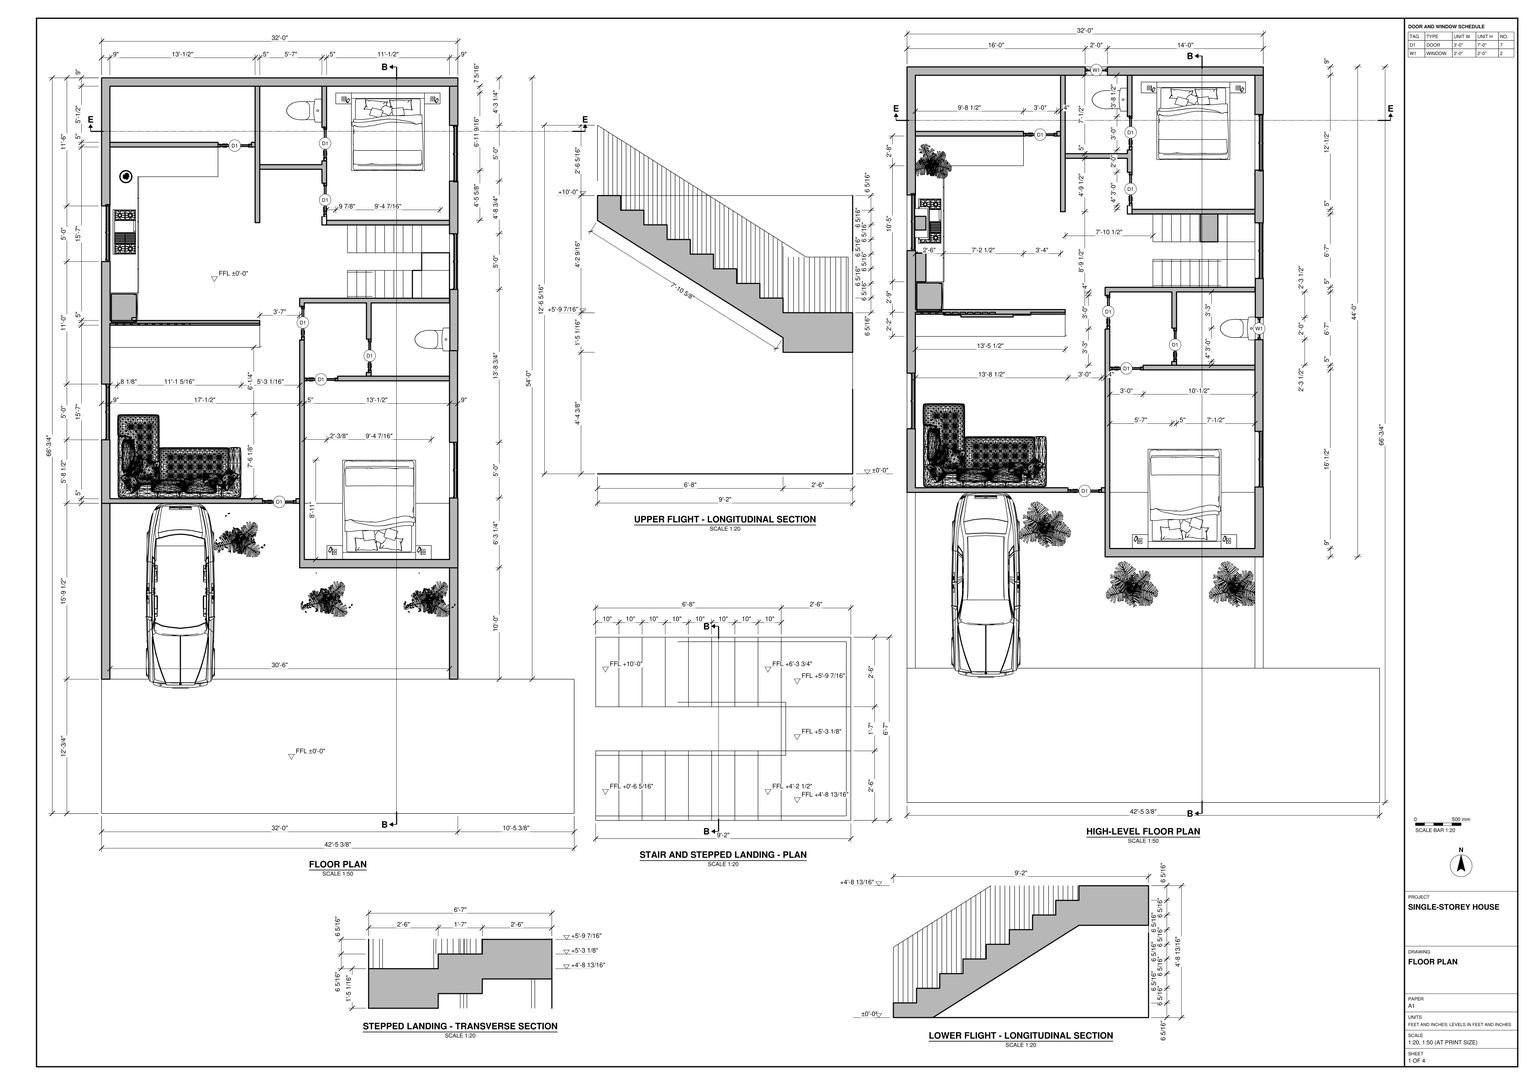
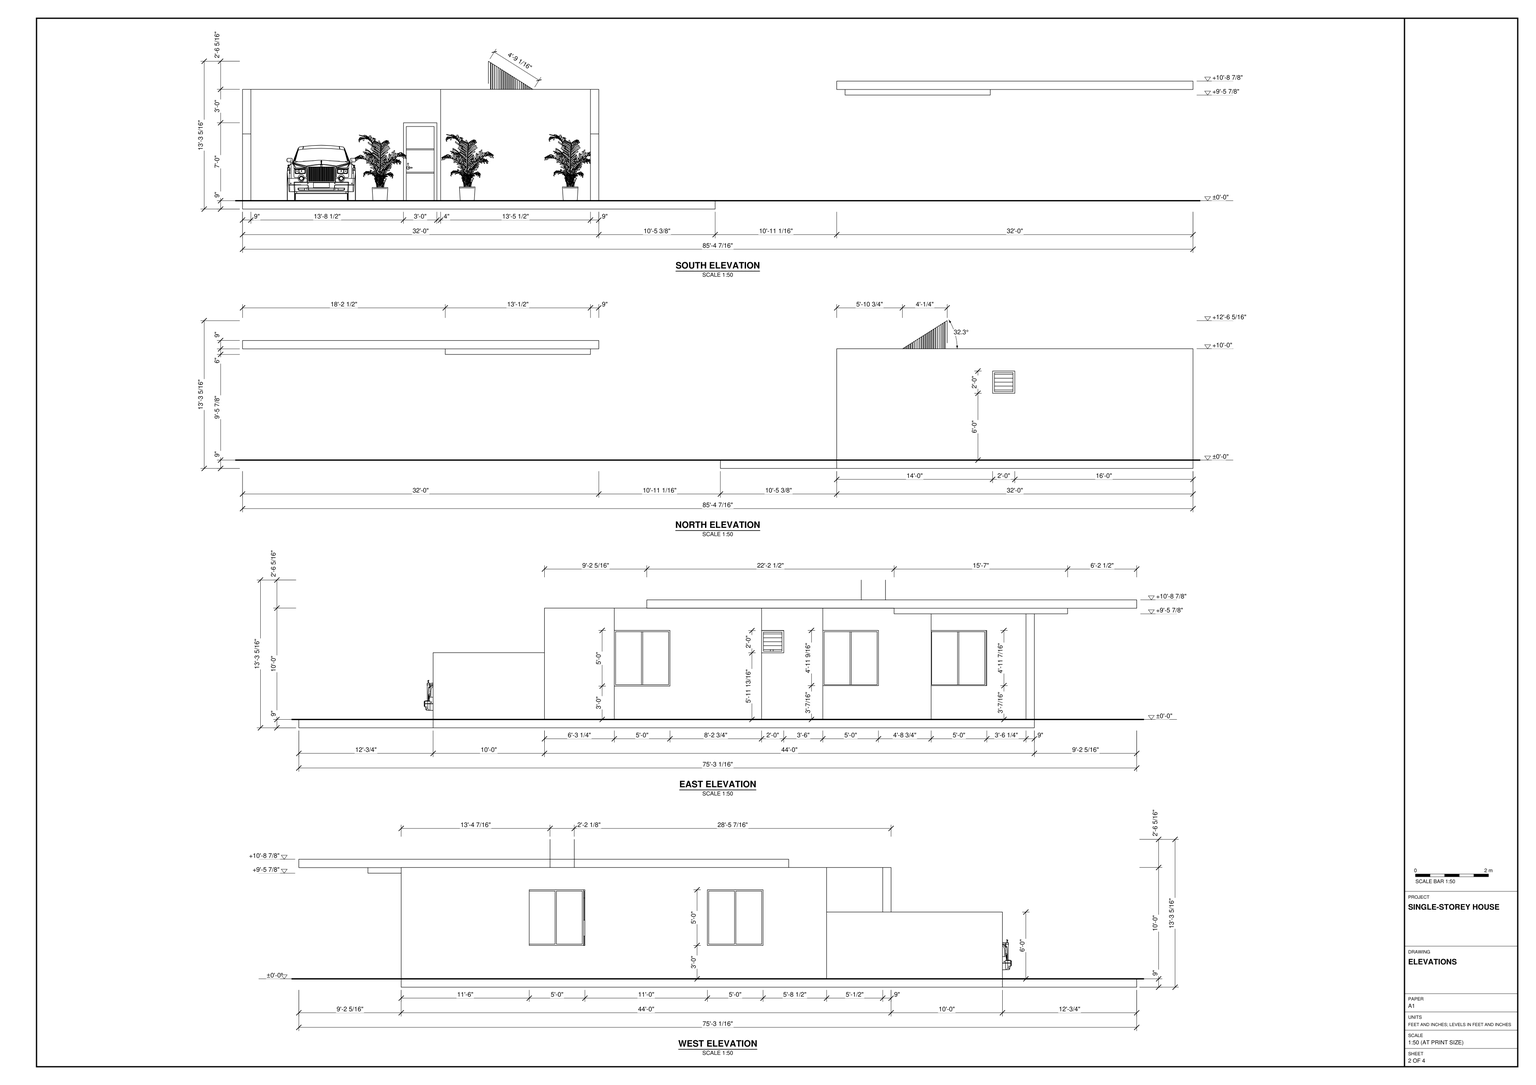
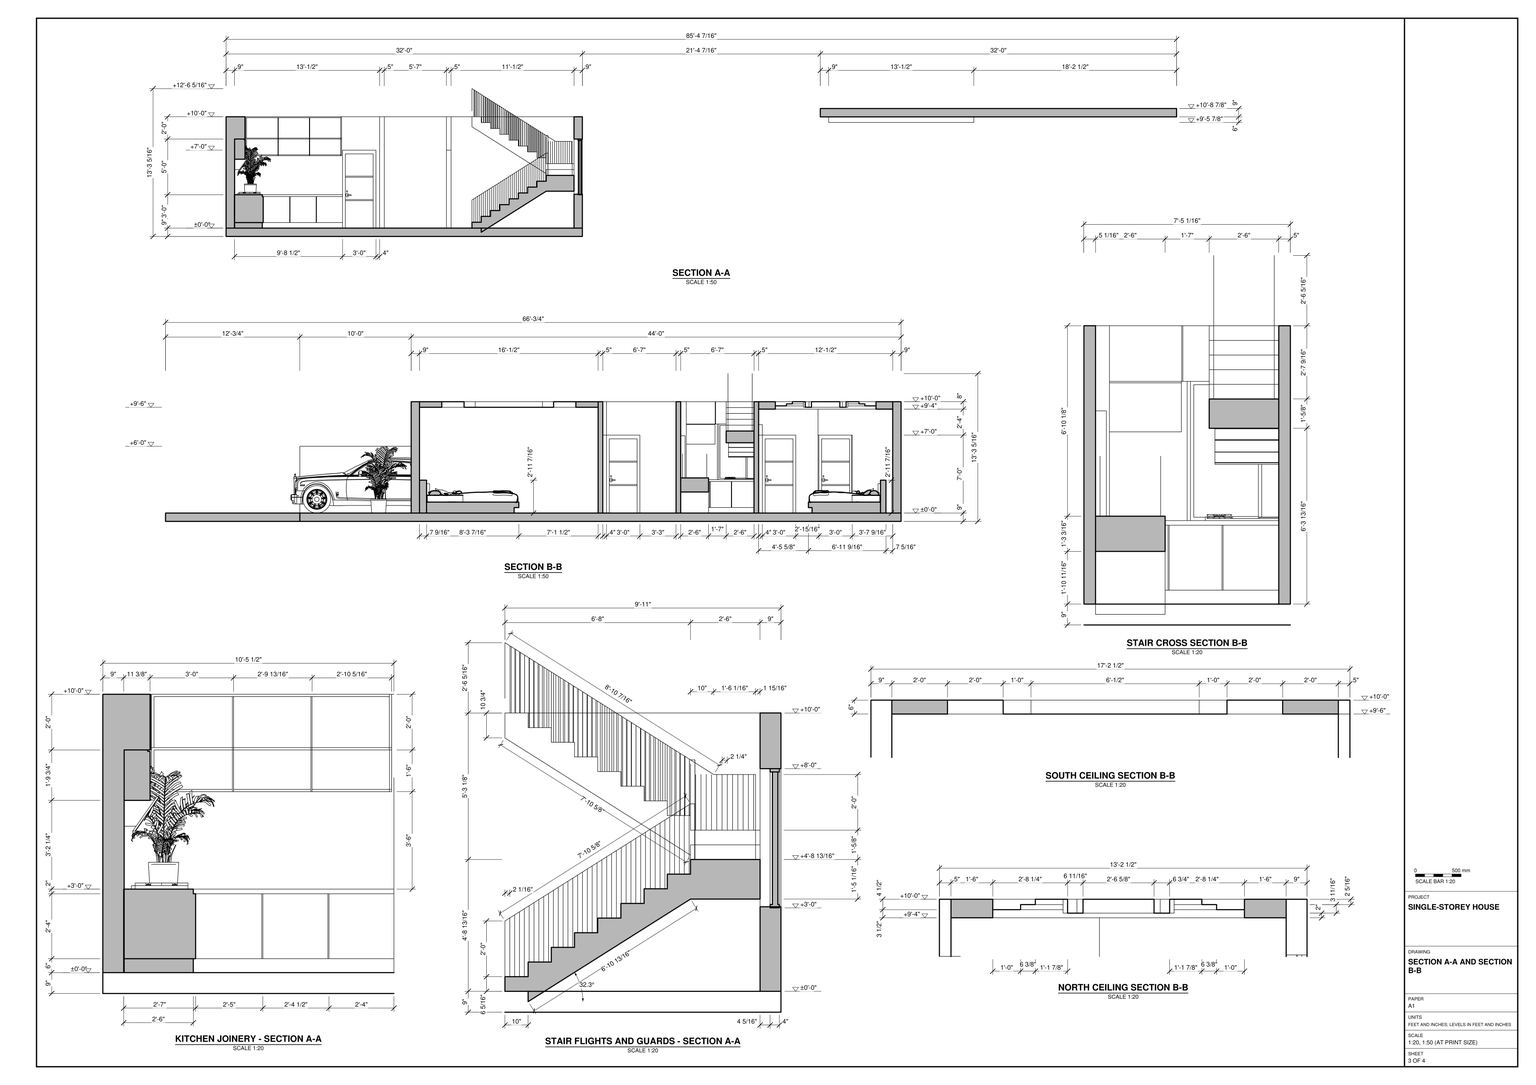
Build the house in SketchUp from task_files/diagram_01.pdf. Work in feet and inches. Set the single ground-floor level to ±0'-0". The overall model extents, including the forecourt and the separately positioned roof slab, are 85'-4 7/16" along X, 75'-3 1/16" along Y and 11'-5 7/8" along Z.

Lay out the 32'-0" wide house with the parking forecourt to the south. Model the floor slab, forecourt walls, 9" exterior walls and interior partitions at their drawn thicknesses. Place the living area in front of the kitchen on the west side, with bedrooms at opposite ends of the east side. Follow the plans for the toilet compartments, connecting spaces, doors, side windows and high-level vents. Build the return stair between the bedrooms with two parallel flights, a stepped landing and guards. Follow the ceiling profiles in section and position the flat roof slab east of the house as shown in the elevations.

Model the kitchen counters, base cabinets and wall cabinets. Size and orient the beds, bedside units and corner sofa to match their plan footprints. Include the cooktop, toilet fixtures, parked car and planting in the positions shown. Decor and loose items may be any suitable library components.

Keep shell elements such as walls, slabs and roof, and each furniture or joinery piece, in separate groups or components. Use components for repeated parts. Save one SketchUp model as output_files/single_storey_house_with_its_stair_and_offset_roof_slab.skp.

# SketchUp Ruby script. Lengths in inches.
U = 1.inch
M = Sketchup.active_model
def pt(a) = Geom::Point3d.new(a.map { |v| v * U })
def face(e, loops, mat)
  f = e.add_face(loops[0].map { |a| pt(a) })
  loops[1..].each { |l| e.add_face(l.map { |a| pt(a) }).erase! }
  f.material = f.back_material = mat if mat
  f
end
# faces: each face lists its corners as indices into pts; further lists are holes
def faces(e, pts, list, mat = nil) = list.each { |f| face(e, (f[0].is_a?(Array) ? f : [f]).map { |l| l.map { |i| pts[i] } }, mat) }
# xy, xz, yz: faces in a plane at the given z, y or x. An outline is a flat list of corners, or four numbers for a rectangle; further outlines are holes
def ring(l) = l.size == 4 ? [[l[0], l[1]], [l[2], l[1]], [l[2], l[3]], [l[0], l[3]]] : l.each_slice(2).to_a
def flat(e, list, mat, &to3) = list.each { |f| face(e, (f[0].is_a?(Array) ? f : [f]).map { |l| ring(l).map { |u, v| to3.(u, v) } }, mat) }
def xy(e, z, list, mat = nil) = flat(e, list, mat) { |x, y| [x, y, z] }
def xz(e, y, list, mat = nil) = flat(e, list, mat) { |x, z| [x, y, z] }
def yz(e, x, list, mat = nil) = flat(e, list, mat) { |y, z| [x, y, z] }
def lines(e, pts, list) = list.each { |a, b| e.add_line(pt(pts[a]), pt(pts[b])) }
# prism: a flat outline (further loops are holes) pulled along v
def prism(e, loops, v, mat = nil)
  f = face(e, loops, mat); d = Geom::Vector3d.new(v.map { |x| x * U })
  f.pushpull(f.normal.samedirection?(d) ? d.length : -d.length)
end
def box(e, o, s, mat = nil) = prism(e, [[o, [o[0] + s[0], o[1], o[2]], [o[0] + s[0], o[1] + s[1], o[2]], [o[0], o[1] + s[1], o[2]]]], [0, 0, s[2]], mat)
def at(x, y, z, deg = 0) = Geom::Transformation.translation(pt([x, y, z])) * Geom::Transformation.rotation(ORIGIN, Z_AXIS, deg.degrees)
def axes(o, x, y, z) = Geom::Transformation.new([*x, 0, *y, 0, *z, 0, *pt(o).to_a, 1])
def part(name) = M.definitions.add(name)
# library, detail: a bought-in or finely detailed component or shape, given as its bounding box
def library(name, o, s) = part(name).tap { |d| box(d.entities, o, s) }
def detail(e, o, s) = box(e.add_group.entities, o, s)
def put(e, d, t, mat = nil) = e.add_instance(d, t).tap { |i| i.material = mat if mat }
def group(e, t, mat = nil) = e.add_group.tap { |g| g.transformation = t; g.material = mat if mat }.entities
root = M.entities
M.materials.add("[Blacktop New]").color = [30, 30, 30]
M.materials.add("[Brick Tumbled]").color = [135, 132, 132]
M.materials.add("[Carrera Marble]").color = [207, 207, 207]
M.materials.add("[Color B08]").color = [102, 25, 0]
M.materials.add("[Color C01]").color = [255, 229, 204]
M.materials.add("[Color C08]").color = [102, 51, 0]
M.materials.add("[Color D07]").color = [153, 114, 0]
M.materials.add("[Color I02]").color = [153, 153, 255]
M.materials.add("[Color I08]").color = [0, 0, 102]
M.materials.add("[Color M09]").color = [0, 0, 0]
M.materials.add("[Color_008]").color = [30, 30, 30]
M.materials.add("[Color_009]").color = [0, 0, 0]
M.materials.add("[Roofing Scalloped]").color = [186, 138, 96]
M.materials.add("[Translucent Glass Gray]").color = [128, 128, 128]
M.materials["[Translucent Glass Gray]"].alpha = 0.5
M.materials.add("[Translucent Glass Tinted]1").color = [7, 201, 240]
M.materials["[Translucent Glass Tinted]1"].alpha = 0.48
M.materials.add("[Translucent_Glass_Gray]").color = [128, 128, 128]
M.materials["[Translucent_Glass_Gray]"].alpha = 0.5
M.materials.add("[Wood Cherry Original]").color = [152, 86, 42]
M.materials.add("[Wood Floor Parquet]").color = [145, 89, 39]
M.materials.add("[Wood Floor]").color = [155, 105, 61]
c1 = library("main+door",[0,-0.79,0],[47.24,7.88,82.68])
c2 = library("Gas cooktop",[0,0,34.52],[24.41,48.07,2.63])
c3 = part("Inclined chimney")
g1 = group(c3.entities,at(1.97,2.08,2.89))
xy(g1,0,[[0,7.9,31.3,13.68]])
xy(g1,11.29,[[0,0,31.3,13.68]])
xz(g1,13.68,[[0,0,31.3,11.29]])
yz(g1,0,[[7.9,0,0,11.29,13.68,11.29,13.68,0]])
yz(g1,31.3,[[7.9,0,13.68,0,13.68,11.29,0,11.29]])
g2 = group(c3.entities,at(0,9.85,0.4))
g3 = group(g2,at(0,0.61,0.43))
prism(g3,[[[35.24,0,0],[35.24,-3.39,4.84],[35.24,-3.58,4.7],[35.24,-0.29,0]]],[-35.24,0,0])
g4 = group(g2,at(0,-3.21,4.99))
prism(g4,[[[35.24,-0.2,-0.12],[35.24,-3.16,5],[0,-3.16,5],[0,-0.2,-0.12]]],[0,0.2,0.12])
g5 = group(g2,at(0,-6.27,10.27))
prism(g5,[[[35.24,-0.19,-0.14],[35.24,-3.58,4.7],[0,-3.58,4.7],[0,-0.19,-0.14]]],[0,0.19,0.14])
g6 = group(g2,at(0,0.61,0.43))
prism(g6,[[[35.24,0,0],[35.24,0.96,0],[35.24,-9.52,14.96],[35.24,-10.16,14.51]]],[-35.24,0,0])
g7 = group(c3.entities,at(10.24,3.95,20.8))
box(g7,[0,0,-6.62],[14.76,11.8125,20.56])
g8 = group(c3.entities,at(0,10.1,0))
prism(g8,[[[35.24,0.46,0],[35.24,1.33,0],[35.24,1.33,0.83],[35.24,1.01,0.83],[35.24,0.37,0.83],[35.24,0,0.83],[35.24,0,0.64]]],[-35.24,0,0])
c4 = part("Inclined+chimney")
put(c4.entities,c3,at(34.17,38.97,0.69))
c5 = library("Component\#33",[0,0,0],[60.64,55.48,158.625])
c6 = library("CS300DRT",[0,0,0],[27.18,17.85,30.31])
c7 = library("Senza",[-40.91,-66.2,-0.5],[133.3,90.15,38.26])
c8 = library("Double bed",[0,0,0],[83.59,112.46,35.43])
c9 = library("RR Phanton",[0,0,0],[8.78,23.57,7.05])
c10 = library("SKT_Nearly Natural 5' Kentia Palm Silk Tree",[-23.18,-17.61,0],[47.48,43.95,59.125])
c11 = library("Group\#5",[0,0,-4.44],[132.5,79,154.74])
c12 = part("Component\#1")
xy(c12.entities,0,[[0,-2,6.1875,0]])
xy(c12.entities,88,[[0,-2,6.1875,0]])
xz(c12.entities,-2,[[0,0,6.1875,88]],"[Color I02]")
xz(c12.entities,0,[[0,0,6.1875,88]])
yz(c12.entities,0,[[-2,0,0,88]])
yz(c12.entities,6.1875,[[-2,0,0,88]])
c13 = part("ventilator")
g9 = group(c13.entities,at(0,0,0))
xy(g9,0,[[0,0,24,1],[0,1,24,6.83]],"[Wood Floor Parquet]")
xy(g9,1.75,[[2,0,22,6.83]],"[Wood Floor Parquet]")
xy(g9,21.87,[[2,0,22,6.83]],"[Wood Cherry Original]")
xy(g9,23.62,[[0,0,24,1],[0,1,24,6.83]],"[Wood Floor Parquet]")
xz(g9,0,[[[0,0,24,23.62],[2,1.75,22,21.87]]],"[Wood Floor Parquet]")
xz(g9,6.83,[[[0,0,24,23.62],[2,1.75,22,21.87]]],"[Wood Cherry Original]")
yz(g9,0,[[0,0,1,23.62],[1,0,6.83,23.62]],"[Wood Floor Parquet]")
yz(g9,2,[[0,1.75,6.83,1.75,6.83,7.66,0,3.5],[0,3.5,6.83,7.66,6.83,11.8125,0,7.66],[0,7.66,6.83,11.8125,6.83,15.97,0,11.8125],[0,11.8125,6.83,15.97,6.83,20.12,0,15.97],[0,15.97,6.83,20.12,6.83,21.87,0,21.87]],"[Wood Floor Parquet]")
yz(g9,22,[[0,1.75,0,3.5,6.83,7.66,6.83,1.75],[0,3.5,0,7.66,6.83,11.8125,6.83,7.66],[0,7.66,0,11.8125,6.83,15.97,6.83,11.8125],[0,11.8125,0,15.97,6.83,20.12,6.83,15.97],[0,15.97,0,21.87,6.83,21.87,6.83,20.12]],"[Wood Floor Parquet]")
yz(g9,24,[[0,0,1,23.62],[1,0,6.83,23.62]],"[Wood Floor Parquet]")
p = [[2,0,3.5],[2,6.83,7.66],[22,6.83,7.66],[22,0,3.5],[2,6.83,11.8125],[2,0,7.66],
  [22,0,7.66],[22,6.83,11.8125],[2,0,11.8125],[2,6.83,15.97],[22,6.83,15.97],[22,0,11.8125],
  [2,6.83,20.12],[2,0,15.97],[22,0,15.97],[22,6.83,20.12]]
faces(g9,p,[[0,1,2,3],[4,5,6,7],[8,9,10,11]],"[Translucent Glass Tinted]1")
faces(g9,p,[[12,13,14,15]],"[Translucent Glass Gray]")
c14 = part("Group\#2")
xy(c14.entities,0,[[0,0,82.68,1.18]],"[Color_009]")
xy(c14.entities,1.97,[[1.97,0.98,40.35,1.18],[42.32,0.98,80.71,1.18]])
xy(c14.entities,1.97,[[1.97,0,40.35,0.3],[42.32,0,80.71,0.3]],"[Color_009]")
xy(c14.entities,80.71,[[1.97,0,40.35,0.3],[42.32,0,80.71,0.3],[1.97,0.3,40.35,0.98],[42.32,0.3,80.71,0.98],[1.97,0.98,40.35,1.18],
  [42.32,0.98,80.71,1.18]])
xy(c14.entities,82.68,[[0,0,82.68,1.18]],"[Color_008]")
xz(c14.entities,0,[[[0,0,82.68,82.68],[1.97,1.97,40.35,80.71],[42.32,1.97,80.71,80.71]]],"[Color_009]")
xz(c14.entities,0.3,[[1.97,1.97,40.35,80.71],[42.32,1.97,80.71,80.71]],"[Translucent_Glass_Gray]")
xz(c14.entities,0.98,[[1.97,1.97,40.35,80.71],[42.32,1.97,80.71,80.71]],"[Translucent_Glass_Gray]")
xz(c14.entities,1.18,[[[0,0,82.68,82.68],[1.97,1.97,80.71,80.71]],[40.35,1.97,42.32,80.71]],"[Color_009]")
yz(c14.entities,0,[[0,0,1.18,82.68]],"[Color_009]")
yz(c14.entities,1.97,[[0.98,1.97,1.18,80.71]])
yz(c14.entities,1.97,[[0,1.97,0.3,80.71]],"[Color_009]")
yz(c14.entities,40.35,[[0,1.97,0.3,80.71],[0.98,1.97,1.18,80.71]],"[Color_009]")
yz(c14.entities,42.32,[[0,1.97,0.3,80.71],[0.98,1.97,1.18,80.71]])
yz(c14.entities,80.71,[[0,1.97,0.3,80.71],[0.98,1.97,1.18,80.71]],"[Color_009]")
yz(c14.entities,82.68,[[0,0,1.18,82.68]],"[Color_009]")
xy(root,-9,[[0,0,509.375,144.75]])
xy(root,0,[[0,0,509.375,144.75]],"[Blacktop New]")
xy(root,0,[[9,144.75,9,334.25,384,334.25,384,264.75,375,264.75,375,144.75]],"[Roofing Scalloped]")
xy(root,6,[[9,561.25,9,718.25,39,718.25,39,688.25,40,688.25,40,663.35,39,663.35,39,662.85,40,662.85,40,637.95,39,637.95,39,637.45,40,637.45,40,610.25,39,610.25,39,609.75,40,609.75,40,587,39,587,39,586.5,40,586.5,40,561.25],[40,687.25,40,688.25,39,688.25,39,718.25,125.5,718.25,125.5,687.25,97.5,687.25,97.5,688.25,97,688.25,97,687.25,69,687.25,69,688.25,68.5,688.25,68.5,687.25]])
xy(root,34,[[39,561.25,40,586.5],[39,587,40,609.75],[39,610.25,40,637.45],[39,637.95,40,662.85],[39,663.35,40,686.25],
  [40,686.25,40,687.25,68.5,687.25,68.5,688.25,69,688.25,69,687.25,97,687.25,97,688.25,97.5,688.25,97.5,687.25,125.5,687.25,125.5,686.25]])
xy(root,36,[[9,561.25,39,561.25,39,686.25,125.5,686.25,125.5,718.25,9,718.25]],"[Carrera Marble]")
xy(root,72,[[0,144.75,9,334.25],[375,144.75,384,264.75]],"[Roofing Scalloped]")
xy(root,74.25,[[9.1875,561.25,20.375,592.25]])
xy(root,95.375,[[19.375,561.25,20.375,592.25]])
xy(root,96,[[9.1875,561.25,19.375,592.25]])
xz(root,0,[[0,-9,509.375,0]],"[Blacktop New]")
xz(root,144.75,[[0,-9,509.375,0]])
xz(root,144.75,[[0,0,9,72],[375,0,384,72]],"[Roofing Scalloped]")
xz(root,264.75,[[375,0,384,72]],"[Roofing Scalloped]")
xz(root,334.25,[[0,0,9,72]],"[Roofing Scalloped]")
xz(root,561.25,[[9,6,40,6,40,34,39,34,39,36,9,36],[9.1875,74.25,20.375,74.25,20.375,95.375,19.375,95.375,19.375,96,9.1875,96]])
xz(root,586.5,[[39,6,40,34]])
xz(root,587,[[39,6,40,34]])
xz(root,592.25,[[9.1875,74.25,9.1875,96,19.375,96,19.375,95.375,20.375,95.375,20.375,74.25]])
xz(root,609.75,[[39,6,40,34]])
xz(root,610.25,[[39,6,40,34]])
xz(root,637.45,[[39,6,40,34]])
xz(root,637.95,[[39,6,40,34]])
xz(root,662.85,[[39,6,40,34]])
xz(root,663.35,[[39,6,40,34]])
xz(root,686.25,[[39,34,125.5,36]])
xz(root,687.25,[[40,6,68.5,34],[69,6,97,34],[97.5,6,125.5,34]],"[Wood Floor]")
xz(root,688.25,[[68.5,6,69,34],[97,6,97.5,34]])
xz(root,718.25,[[9,6,39,36],[39,6,125.5,36]])
yz(root,0,[[0,-9,144.75,0]],"[Blacktop New]")
yz(root,0,[[144.75,0,334.25,72]],"[Roofing Scalloped]")
yz(root,9,[[561.25,6,718.25,36]])
yz(root,9,[[144.75,0,334.25,72]],"[Roofing Scalloped]")
yz(root,9.1875,[[561.25,74.25,592.25,96]])
yz(root,19.375,[[561.25,95.375,592.25,96]])
yz(root,20.375,[[561.25,74.25,592.25,95.375]],"[Wood Floor Parquet]")
yz(root,39,[[586.5,6,587,34],[609.75,6,610.25,34],[637.45,6,637.95,34],[662.85,6,663.35,34]])
yz(root,39,[[561.25,34,686.25,36]],"[Carrera Marble]")
yz(root,40,[[561.25,6,586.5,34],[587,6,609.75,34],[610.25,6,637.45,34],[637.95,6,662.85,34],[663.35,6,687.25,34]],"[Wood Floor]")
yz(root,68.5,[[687.25,6,688.25,34]])
yz(root,69,[[687.25,6,688.25,34]])
yz(root,97,[[687.25,6,688.25,34]])
yz(root,97.5,[[687.25,6,688.25,34]])
yz(root,125.5,[[687.25,6,718.25,6,718.25,36,686.25,36,686.25,34,687.25,34]],"[Wood Floor]")
yz(root,375,[[144.75,0,264.75,72]],"[Roofing Scalloped]")
yz(root,384,[[144.75,0,264.75,72]],"[Roofing Scalloped]")
yz(root,509.375,[[0,-9,144.75,0]],"[Blacktop New]")
# 378 loose lines left out
p = [[1.77,722.75,0],[9,718.25,0],[9,718.25,6],[1.77,722.75,6]]
faces(root,p,[[0,1,2,3]])
put(root,c1,axes([218.5,466.25,0],[0.762,0,0],[0,0.5,0],[0,0,1.016]))
put(root,c2,at(12.3,602.59,1.48))
put(root,c4,at(63.3,572.56,59.53,90))
put(root,c5,axes([38.29,529.61,3.99],[0,0.5,0],[-0.5,0,0],[0,0,0.5]))
put(root,c6,axes([375.36,523.28,0],[-1.39,0,0],[0,-1.39,0],[0,0,1.39]))
put(root,c7,at(109.53,363.83,0.5,180))
put(root,c8,at(364.86,692.87,0,90))
put(root,c8,axes([242.9,380.75,0],[0,-1.28,0],[1,0,0],[0,0,1]))
put(root,c6,axes([237.1875,769.86,0],[-1.39,0,0],[0,-1.39,0],[0,0,1.39]))
put(root,c9,axes([47.71,135.0625,0],[8.4825,0,0],[0,8.4825,0],[0,0,8.4825]))
put(root,c10,axes([242.16,229.53,0],[1.29,0,0],[0,1.29,0],[0,0,1.29]))
put(root,c10,axes([353.16,229.53,0],[1.29,0,0],[0,1.29,0],[0,0,1.29]))
put(root,c10,axes([148.125,293.89,-0.68],[1.29,0,0],[0,1.29,0],[0,0,1.29]))
put(root,c10,at(26.15,686.21,36))
g10 = group(root,at(0,264.75,-9))
box(g10,[0,-120,0],[384,648,9])
put(root,c11,at(242.5,555.25,0))
g11 = group(root,at(9,502.25,0))
xz(g11,26,[[6.1875,32,8,120]])
g12 = group(g11,at(0,26,0))
xy(g12,0,[[0,-26,161.5,0]])
xy(g12,6,[[0,-26,161.5,-24]],"[Wood Floor]")
xy(g12,8,[[54.5,-25,106.5,-24],[107,-25,159.5,-24]])
xy(g12,8,[[2,-24,54,0]],"[Color I02]")
xy(g12,18,[[2,-25,5.55,0],[5.55,-25,54,0]],"[Color I02]")
xy(g12,18.5,[[2,-25,54,0]],"[Color I02]")
xy(g12,28,[[54.5,-25,106.5,-24],[107,-25,159.5,-24]])
xy(g12,28,[[2,-24,54,0]],"[Color I02]")
xy(g12,30,[[0,-26,161.5,-24]])
xy(g12,32,[[0,-26,161.5,0]],"[Wood Floor]")
xy(g12,50.05,[[30.78,-3,124.35,0]])
xy(g12,60.92,[[49.14,-5,105.39,-3]],"[Color M09]")
xy(g12,90.67,[[49.14,-5,105.39,-3]],"[Color M09]")
xy(g12,102.3,[[30.78,-3,124.35,0]])
xy(g12,103.52,[[14.625,-21,143.0625,0]],"[Wood Floor]")
xy(g12,104.38,[[14.625,-21,143.0625,0]],"[Wood Floor]")
xz(g12,-26,[[0,0,161.5,6],[0,30,161.5,32]],"[Wood Floor]")
xz(g12,-25,[[54.5,8,106.5,18],[107,8,159.5,18],[54.5,18.5,106.5,28],[107,18.5,159.5,28]],"[Color I02]")
xz(g12,-25,[[2,18,54,18.5],[54.5,18,106.5,18.5],[107,18,159.5,18.5]],"[Wood Floor]")
xz(g12,-24,[[106.5,8,107,28]])
xz(g12,-24,[[[0,6,161.5,30],[2,8,159.5,28]],[54,8,54.5,28]],"[Wood Floor]")
xz(g12,-21,[[14.625,103.52,143.0625,104.38]],"[Wood Floor]")
xz(g12,-5,[[49.14,60.92,105.39,90.67]],"[Color M09]")
xz(g12,-3,[[[30.78,50.05,124.35,102.3],[49.14,60.92,105.39,90.67]]])
xz(g12,0,[[[8,32,161.5,120],[30.78,50.05,124.35,102.3],[14.625,103.52,143.0625,104.38]]])
xz(g12,0,[[2,8,54,18],[2,18.5,54,28]],"[Color I02]")
yz(g12,0,[[-26,0,0,6],[-24,6,0,30],[-26,30,0,32]],"[Wood Floor]")
yz(g12,2,[[-25,18,-24,18.5]])
yz(g12,2,[[-24,8,0,18],[-24,18.5,0,28]],"[Color I02]")
yz(g12,14.625,[[-21,103.52,0,104.38]],"[Wood Floor]")
yz(g12,30.78,[[-3,50.05,0,102.3]])
yz(g12,49.14,[[-5,60.92,-3,90.67]],"[Color M09]")
yz(g12,54,[[-25,18,-24,18.5]])
yz(g12,54,[[-24,8,0,18],[-24,18.5,0,28]],"[Color I02]")
yz(g12,54.5,[[-25,8,-24,28]])
yz(g12,105.39,[[-5,60.92,-3,90.67]],"[Color M09]")
yz(g12,106.5,[[-25,8,-24,28]])
yz(g12,107,[[-25,8,-24,28]])
yz(g12,124.35,[[-3,50.05,0,102.3]])
yz(g12,143.0625,[[-21,103.52,0,104.38]],"[Wood Floor]")
yz(g12,159.5,[[-25,8,-24,28]])
yz(g12,161.5,[[-26,0,0,6],[-24,6,0,30],[-26,30,0,32]],"[Wood Floor]")
# 6 loose lines left out
put(g12,c12,at(0,0,32),"[Color I08]")
put(g12,c12,at(8,0,32))
put(g12,c12,at(16,0,32))
put(g12,c12,at(24,0,32))
put(g12,c12,at(32,0,32))
put(g12,c12,at(40,0,32))
put(g12,c12,at(48,0,32))
put(g12,c12,at(56,0,32))
put(g12,c12,at(64,0,32))
put(g12,c12,at(72,0,32))
put(g12,c12,at(80,0,32))
g13 = group(root,at(9,531.25,0),"[Wood Floor]")
xy(g13,0,[[0,0,0,187,116.5,187,116.5,157,30,157,30,0]])
xy(g13,6,[[0,0,30,0,30,157,116.5,157,116.5,187,0,187]])
xz(g13,0,[[0,0,30,6]])
xz(g13,157,[[30,0,116.5,6]],"[Carrera Marble]")
xz(g13,187,[[0,0,116.5,6]])
yz(g13,0,[[0,0,187,6]])
yz(g13,30,[[0,0,157,6]],"[Carrera Marble]")
yz(g13,116.5,[[157,0,187,6]])
# 1 loose lines left out
g14 = group(root,at(0,264.75,0),"[Color C01]")
xy(g14,0,[[213.5,9,218.5,245.5],[0,69.5,9,198],[209.5,69.5,213.5,74.5],[375,75.25,383.64,234.01],[254.5,201.5,375,206.5],
  [285.3125,206.5,290.5,210.5],[375.36,234.01,384,300],[285.5,246.5,290.5,285.5],[9,266.5,9.1875,330],[375,300,384,416.75],
  [0,330,9.1875,390],[237.5,369.5,242.5,378.5],[242.5,369.5,375,374.5],[165.5,372,170.5,519],[0,390,0,519,9,519,9,453.5,9.0625,453.5,9.0625,390],
  [375,416.75,384,519],[9,453.5,125.5,458.5],[161.5,453.5,165.5,458.5],[237.5,474.5,242.5,519],[0,519,216,528],
  [216,519,384,528]])
xy(g14,36,[[375,75.25,383.64,135.25],[0,138,9,198],[0,330,9.1875,390]])
xy(g14,36.45,[[375,300,384,360],[375,416.75,384,476.75]])
xy(g14,71.79,[[375.36,234.01,384,257.99]])
xy(g14,72,[[192.02,519,216,528]])
xy(g14,78,[[21.04,435.39,22.04,435.39,56.37,435.43,89.69,435.46,124.52,435.5,124.5,453.5,21.02,453.39]])
xy(g14,79,[[22.04,434.39,55.87,435.39],[90.19,434.39,123.59,435.39],[56.37,435.39,56.37,435.43,89.69,435.46],[56.37,435.43,56.3,465.26,89.63,465.34,89.69,435.46]])
xy(g14,84,[[173.5,69.5,209.5,74.5],[218.5,201.5,254.5,206.5],[285.5,206.5,290.5,246.5],[213.5,245.5,218.5,281.5],[237.5,369.5,242.5,414.5],
  [237.5,438.5,242.5,474.5],[125.5,453.5,161.5,458.5]])
xy(g14,95.9,[[375,416.75,384,476.75]])
xy(g14,96,[[375,75.25,383.64,135.25],[0,138,9,198],[375.36,234.01,384,257.99],[9.1875,296.5,20.375,327.63],[375,300,384,360],
  [9.1875,327.63,9.1875,330,20.375,330,20.375,328.13,19.375,328.13,19.375,327.63],[0,330,20.375,330,20.375,358.77,19.375,358.77,19.375,359.27,20.375,359.27,20.375,389.9,19.375,389.9,9.0625,390,0,390],[19.375,389.9,19.375,390,9.0625,390],[9.0625,390,9.6875,453.5,21.02,453.39,20.71,421.64,19.6875,421.65,19.375,390],[22.04,434.39,55.87,435.39],
  [90.19,434.39,123.59,435.39],[56.37,435.39,89.69,435.46,89.65,453.46,56.33,453.43,56.37,435.43],[56.33,453.43,89.65,453.46,89.63,465.34,56.3,465.26],[192.02,519,216,528]])
xy(g14,97,[[56.37,434.3,56.37,435.39,89.69,435.39,89.69,434.34],[90.19,434.34,90.19,435.39,123.52,435.39,123.52,434.375],[22.04,434.39,22.04,435.39,55.87,435.39,55.87,434.43],[22.04,435.39,55.87,435.43,55.87,435.39],[55.87,435.39,56.37,435.43],
  [56.37,435.39,56.37,435.43,89.69,435.46,89.69,435.39],[89.69,435.39,90.19,435.46],[90.19,435.39,90.19,435.46,123.52,435.5,123.52,435.39]])
xy(g14,119,[[56.37,434.3,89.69,434.34,89.69,435.46,56.37,435.43],[90.19,434.34,123.52,434.375,123.52,435.5,90.19,435.46],[22.04,434.39,55.87,434.43,55.87,435.43,22.04,435.39]])
xy(g14,120,[[213.5,0,375,0,375,9,218.5,9,218.5,285.5,285.5,285.5,285.5,210.5,290.5,210.5,290.5,285.5,375,285.5,375,290.5,213.5,290.5],[375,0,384,75.25],[0,69.5,9,198],[9,69.5,213.5,74.5],[375,75.25,383.64,234.01],
  [218.5,201.5,375,206.5],[285.3125,206.5,285.5,210.5],[285.5,206.5,290.5,210.5],[375.36,234.01,384,300],[9,261.5,170.5,266.5],
  [375,300,384,416.75],[237.5,369.5,242.5,369.5,242.5,438.5,237.5,438.5,237.5,434.5,170.5,434.5,170.5,429.5,237.5,429.5],[242.5,369.5,375,374.5],[165.5,372,170.5,519],[375,416.75,384,519],
  [237.5,438.5,242.5,519],[9,453.5,165.5,458.5],[0,519,384,528]])
xy(g14,120,[[0,198,9,198,9,266.5,9.1875,266.5,9.1875,296.5,20.375,296.5,20.375,327.63,19.375,327.63,19.375,328.13,20.375,328.13,20.375,358.77,19.375,358.77,19.375,359.27,20.375,359.27,20.375,389.9,19.375,389.9,19.6875,421.65,20.71,421.64,21.02,453.39,9.6875,453.5,9.0625,445.85,9.0625,453.5,9,453.5,9,519,0,519],[21.04,435.39,124.52,435.5,124.5,453.5,9.6875,453.5,21.02,453.39]],"[Wood Floor Parquet]")
xz(g14,0,[[375,0,384,120]])
xz(g14,0,[[213.5,0,375,120]],"[Brick Tumbled]")
xz(g14,9,[[218.5,0,375,120]])
xz(g14,69.5,[[0,0,9,120],[9,0,173.5,0,173.5,84,209.5,84,209.5,0,213.5,0,213.5,120,9,120]])
xz(g14,74.5,[[9,0,173.5,120],[209.5,0,209.5,84,173.5,84,173.5,120,213.5,120,213.5,0]])
xz(g14,75.25,[[383.64,0,383.64,36,375,36,375,96,383.64,96,383.64,120,384,120,384,0]])
xz(g14,135.25,[[375,36,383.64,96]])
xz(g14,138,[[0,36,9,96]])
xz(g14,198,[[0,36,9,96]])
xz(g14,201.5,[[254.5,0,375,0,375,120,218.5,120,218.5,84,254.5,84]])
xz(g14,206.5,[[254.5,0,254.5,84,218.5,84,218.5,120,285.3125,120,285.3125,0],[285.3125,0,290.5,0,290.5,84,285.5,84,285.5,120,285.3125,120],[290.5,0,375,120],[285.5,84,290.5,120]])
xz(g14,210.5,[[285.3125,0,290.5,120]])
xz(g14,234.01,[[375,0,375,120,375.36,120,375.36,96,383.64,96,383.64,71.79,375.36,71.79,375.36,0],[375.36,0,383.64,71.79],[383.64,0,384,71.79],[375.36,96,383.64,120],[383.64,96,384,120]])
xz(g14,245.5,[[213.5,0,218.5,84]])
xz(g14,246.5,[[285.5,0,290.5,84]])
xz(g14,257.99,[[375.36,71.79,384,96]])
xz(g14,261.5,[[9,0,170.5,120]])
xz(g14,266.5,[[9.1875,0,170.5,120]])
xz(g14,281.5,[[213.5,0,218.5,84]])
xz(g14,285.5,[[218.5,0,285.5,120],[290.5,0,375,120]])
xz(g14,290.5,[[213.5,0,218.5,120],[218.5,0,375,120]])
xz(g14,296.5,[[9.1875,96,20.375,120]],"[Wood Floor Parquet]")
xz(g14,300,[[375,0,375.36,36.45],[375.36,0,384,36.45],[375.36,36.45,384,96],[375,96,375.36,120],[375.36,96,384,120]])
xz(g14,327.63,[[19.375,96,20.375,120]])
xz(g14,328.13,[[19.375,96,20.375,120]])
xz(g14,330,[[0,36,9.1875,96]])
xz(g14,358.77,[[19.375,96,20.375,120]])
xz(g14,359.27,[[19.375,96,20.375,120]])
xz(g14,360,[[375,36.45,384,96]])
xz(g14,369.5,[[237.5,0,242.5,84],[242.5,0,375,120],[237.5,84,242.5,120]])
xz(g14,372,[[165.5,0,170.5,120]])
xz(g14,374.5,[[242.5,0,375,120]])
xz(g14,389.9,[[19.375,96,20.375,120]])
xz(g14,390,[[9.0625,0,9.1875,36],[0,36,9.0625,96]])
xz(g14,414.5,[[237.5,0,242.5,84]])
xz(g14,416.75,[[375,36.45,384,95.9]])
xz(g14,429.5,[[170.5,0,237.5,120]])
xz(g14,434.39,[[22.04,79,55.87,96],[90.19,79,123.59,96]],"[Wood Floor Parquet]")
xz(g14,434.5,[[170.5,0,237.5,120]])
xz(g14,435.39,[[22.04,79,55.87,96],[90.19,79,123.59,96],[55.87,96,90.19,97]])
xz(g14,435.43,[[55.87,97,56.37,119]])
xz(g14,435.46,[[89.69,97,90.19,119]])
xz(g14,438.5,[[237.5,0,242.5,84]])
xz(g14,453.5,[[9,0,9.0625,120],[9.0625,0,125.5,0,125.5,84,161.5,84,161.5,0,165.5,0,165.5,120,9.6875,120,9.6875,94.57,9.0625,94.57],[9.0625,94.57,9.6875,120]])
xz(g14,458.5,[[9,0,9,120,165.5,120,165.5,0,161.5,0,161.5,84,125.5,84,125.5,0]])
xz(g14,474.5,[[237.5,0,242.5,84]])
xz(g14,476.75,[[375,36.45,384,95.9]])
xz(g14,519,[[9,0,165.5,120],[165.5,0,170.5,120],[170.5,0,216,0,216,72,192.02,72,192.02,96,216,96,216,120,170.5,120],[216,0,237.5,120],[237.5,0,242.5,120],
  [242.5,0,375,120],[375,0,384,120]])
xz(g14,528,[[[0,0,384,120],[192.02,72,216,96]]])
yz(g14,0,[[[69.5,0,528,120],[330,36,390,96],[138,36,198,96]]])
yz(g14,9,[[74.5,0,198,0,198,36,138,36,138,96,198,96,198,120,74.5,120],[198,0,261.5,120],[453.5,0,458.5,120],[458.5,0,519,120]])
yz(g14,9.0625,[[390,0,453.5,120]])
yz(g14,9.1875,[[266.5,0,390,0,390,36,330,36,330,96,296.5,96,296.5,120,266.5,120]])
yz(g14,19.375,[[327.63,96,328.13,120],[358.77,96,359.27,120]])
yz(g14,20.375,[[296.5,96,327.63,120],[328.13,96,358.77,120],[359.27,96,389.9,120]],"[Wood Floor Parquet]")
yz(g14,22.04,[[434.39,79,435.39,94.38],[434.39,94.38,435.39,96],[434.39,97,435.39,119]])
yz(g14,55.87,[[434.39,79,435.39,79.24],[434.39,79.24,435.39,96],[434.43,97,435.43,119]])
yz(g14,56.37,[[435.39,79,435.43,96],[434.3,97,435.43,119]])
yz(g14,89.69,[[434.34,97,435.46,119]])
yz(g14,90.19,[[434.39,79,435.39,96],[434.34,97,435.46,119]])
yz(g14,123.52,[[434.375,97,435.5,119]])
yz(g14,123.59,[[434.39,79,435.39,96]])
yz(g14,125.5,[[453.5,0,458.5,84]])
yz(g14,161.5,[[453.5,0,458.5,84]])
yz(g14,165.5,[[372,0,453.5,120],[453.5,0,458.5,120],[458.5,0,519,120]])
yz(g14,170.5,[[261.5,0,266.5,120],[372,0,429.5,120],[429.5,0,434.5,120],[434.5,0,519,120]])
yz(g14,173.5,[[69.5,0,74.5,84]])
yz(g14,192.02,[[519,72,528,96]])
yz(g14,209.5,[[69.5,0,74.5,84]])
yz(g14,213.5,[[0,0,9,120],[9,0,69.5,120],[69.5,0,74.5,120],[74.5,0,74.5,120,290.5,120,290.5,0,281.5,0,281.5,84,245.5,84,245.5,0]])
yz(g14,216,[[519,72,528,96]])
yz(g14,218.5,[[9,0,245.5,0,245.5,84,281.5,84,281.5,0,285.5,0,285.5,120,206.5,120,206.5,84,201.5,84,201.5,120,9,120]])
yz(g14,237.5,[[369.5,0,378.5,84],[414.5,0,414.5,84,369.5,84,369.5,120,429.5,120,429.5,0],[434.5,0,438.5,120],[474.5,0,474.5,84,438.5,84,438.5,120,519,120,519,0]])
yz(g14,242.5,[[369.5,0,374.5,84],[374.5,0,378.5,84],[414.5,0,438.5,0,438.5,120,374.5,120,374.5,95.375,378.5,95.375,378.5,84,414.5,84],[474.5,0,519,0,519,120,438.5,120,438.5,84,474.5,84],[369.5,84,374.5,95.375],
  [374.5,84,378.5,95.375],[369.5,95.375,374.5,120]])
yz(g14,254.5,[[201.5,0,206.5,84]])
yz(g14,285.3125,[[206.5,0,210.5,120]])
yz(g14,285.5,[[246.5,0,246.5,84,206.5,84,206.5,120,285.5,120,285.5,0]])
yz(g14,290.5,[[206.5,0,210.5,84],[246.5,0,285.5,0,285.5,120,210.5,120,210.5,84,246.5,84],[206.5,84,210.5,120]])
yz(g14,375,[[9,0,75.25,120],[75.25,0,75.25,36,135.25,36,135.25,96,75.25,96,75.25,120,201.5,120,201.5,0],[201.5,0,206.5,120],[206.5,0,234.01,120],[285.5,0,290.5,120],
  [300,0,300,36.45,360,36.45,360,96,300,96,300,120,369.5,120,369.5,0],[369.5,0,374.5,120],[374.5,0,416.75,120],[416.75,0,416.75,36.45,476.75,36.45,476.75,95.9,416.75,95.9,416.75,120,519,120,519,0]])
yz(g14,375.36,[[234.01,0,234.01,71.79,257.99,71.79,257.99,96,234.01,96,234.01,120,300,120,300,0]])
yz(g14,383.64,[[75.25,0,234.01,0,234.01,120,75.25,120,75.25,96,135.25,96,135.25,36,75.25,36]])
yz(g14,384,[[0,0,75.25,120],[234.01,0,300,0,300,120,234.01,120,234.01,96,257.99,96,257.99,71.79,234.01,71.79],[300,0,416.75,0,416.75,120,300,120,300,96,360,96,360,36.45,300,36.45],[416.75,0,519,0,519,120,416.75,120,416.75,95.9,476.75,95.9,476.75,36.45,416.75,36.45],[519,0,528,120]])
# 16 loose lines left out
p = [[21.04,435.39,78],[22.04,435.39,78],[56.37,435.43,78],[56.37,435.43,79],[56.37,435.43,96],[56.37,435.43,97],
  [55.87,435.43,97],[22.04,435.39,97],[22.04,435.39,119],[55.87,435.43,119],[56.37,435.43,119],[89.69,435.46,119],
  [90.19,435.46,119],[123.52,435.5,119],[123.52,435.5,97],[90.19,435.46,97],[89.69,435.46,97],[89.69,435.46,96],
  [89.69,435.46,79],[89.69,435.46,78],[124.52,435.5,78],[124.52,435.5,120],[21.04,435.39,120],[21.02,453.39,96],
  [21.02,453.39,120],[21.02,453.39,78],[124.5,453.5,120],[124.5,453.5,96],[124.5,453.5,78],[56.33,453.43,96],
  [89.65,453.46,96],[56.3,465.26,79],[56.3,465.26,96],[56.37,435.39,96],[56.37,435.39,79],[89.63,465.34,79],
  [89.63,465.34,96],[4.5,390,120],[4.5,390,96],[4.5,390,94.57],[9.6875,453.5,94.57],[9.6875,453.5,96],
  [9.6875,453.5,120],[9.0625,445.85,120],[19.375,390,96],[19.6875,421.65,96],[19.6875,421.65,120],[19.375,389.9,120],
  [19.375,389.9,96],[20.71,421.64,96],[20.71,421.64,120],[89.69,434.34,119],[56.37,434.3,119],[56.37,434.3,97],
  [89.69,434.34,97],[123.52,434.375,119],[90.19,434.34,119],[90.19,434.34,97],[123.52,434.375,97],[22.04,434.39,97],
  [55.87,434.43,97],[55.87,434.43,119],[22.04,434.39,119]]
faces(g14,p,[[0,1,2,3,4,5,6,7,8,9,10,11,12,13,14,15,16,17,18,19,20,21,22],[23,24,22,0,25],[18,3,2,19],[29,23,25,28,27,30],[31,3,4,29,32],[3,18,17,16,5,4],[17,18,35,36,30],[32,36,35,31],
  [37,38,39,40,41,42,43],[46,45,49,50],[41,42,24,23]])
faces(g14,p,[[26,27,28,20,21],[17,33,34,18],[44,45,46,47,48],[24,50,49,23],[51,52,53,54],[55,56,57,58],[59,60,61,62]],"[Wood Floor Parquet]")
put(g14,c1,axes([125.5,453.5,0],[0.762,0,0],[0,0.5,0],[0,0,1.016]))
put(g14,c1,axes([173.5,69.5,0],[0.762,0,0],[0,0.5,0],[0,0,1.016]))
put(g14,c1,axes([218.5,246.27,0.17],[0,0.762,0],[-0.5,0,0],[0,0,1.016]))
put(g14,c1,axes([242.5,439.4375,0],[0,0.762,0],[-0.5,0,0],[0,0,1.016]))
put(g14,c1,axes([242.5,378.5,0],[0,0.762,0],[-0.5,0,0],[0,0,1.016]))
put(g14,c1,axes([290.5,210.5,0],[0,0.762,0],[-0.5,0,0],[0,0,1.016]))
put(g14,c13,axes([380.6,234.01,71.79],[0,0.99908,0],[-0.33,0,0],[0,0,1.016]))
put(g14,c13,axes([192.02,523.5,72],[0.99908,0,0],[0,0.33,0],[0,0,1.016]))
put(g14,c14,axes([4.5,198,36],[0,-0.72571,0],[3.3988,0,0],[0,0,0.72571]))
put(g14,c14,axes([379.32,360,36],[0,-0.72571,0],[3.3988,0,0],[0,0,0.72571]))
put(g14,c14,axes([379.32,135.25,36],[0,-0.72571,0],[3.3988,0,0],[0,0,0.72571]))
put(g14,c14,axes([379.32,475.9375,36],[0,-0.72571,0],[3.3988,0,0],[0,0,0.72571]))
put(g14,c14,axes([4.5,391.43,36],[0,-0.72571,0],[3.3988,0,0],[0,0,0.72571]))
g15 = group(root,at(9,339.25,114))
xy(g15,0,[[[0,0,204.5,189],[20.07,20.07,184.43,168.93]],[[36,36,168.5,153],[43.36,43.36,161.14,145.64]],[[65.23,65.23,139.27,123.77],[76.08,76.08,128.42,112.92]]],"[Color D07]")
xy(g15,6,[[[0,0,204.5,189],[20.07,20.07,184.43,168.93]],[[20.07,20.07,184.43,168.93],[24,24,180.5,165]],[[24,24,180.5,165],[36,36,168.5,153]],[[43.36,43.36,161.14,145.64],[65.23,65.23,139.27,123.77]],[76.08,76.08,128.42,112.92]])
xz(g15,0,[[0,0,204.5,6]])
xz(g15,20.07,[[20.07,0,184.43,6]])
xz(g15,36,[[36,0,168.5,6]])
xz(g15,43.36,[[43.36,0,161.14,6]])
xz(g15,65.23,[[65.23,0,139.27,6]],"[Color D07]")
xz(g15,76.08,[[76.08,0,128.42,6]],"[Color D07]")
xz(g15,112.92,[[76.08,0,128.42,6]],"[Color D07]")
xz(g15,123.77,[[65.23,0,139.27,6]],"[Color D07]")
xz(g15,145.64,[[43.36,0,161.14,6]])
xz(g15,153,[[36,0,168.5,6]])
xz(g15,168.93,[[20.07,0,184.43,6]])
xz(g15,189,[[0,0,204.5,6]])
yz(g15,0,[[0,0,189,6]])
yz(g15,20.07,[[20.07,0,168.93,6]])
yz(g15,36,[[36,0,153,6]])
yz(g15,43.36,[[43.36,0,145.64,6]])
yz(g15,65.23,[[65.23,0,123.77,6]],"[Color D07]")
yz(g15,76.08,[[76.08,0,112.92,6]],"[Color D07]")
yz(g15,128.42,[[76.08,0,112.92,6]])
yz(g15,139.27,[[65.23,0,123.77,6]],"[Color D07]")
yz(g15,161.14,[[43.36,0,145.64,6]])
yz(g15,168.5,[[36,0,153,6]])
yz(g15,184.43,[[20.07,0,168.93,6]])
yz(g15,204.5,[[0,0,189,6]])
g16 = group(root,at(218.5,273.75,114))
xy(g16,0,[[[0,0,156.5,192.5],[24,24,132.5,168.5]],[[48,48,108.5,144.5],[60,60,96.5,132.5]]])
xy(g16,6,[[[0,0,156.5,192.5],[24,24,132.5,168.5]],[[24,24,132.5,168.5],[48,48,108.5,144.5]],[60,60,96.5,132.5]])
xz(g16,0,[[0,0,156.5,6]])
xz(g16,24,[[24,0,132.5,6]])
xz(g16,48,[[48,0,108.5,6]])
xz(g16,60,[[60,0,96.5,6]])
xz(g16,132.5,[[60,0,96.5,6]])
xz(g16,144.5,[[48,0,108.5,6]])
xz(g16,168.5,[[24,0,132.5,6]])
xz(g16,192.5,[[0,0,156.5,6]])
yz(g16,0,[[0,0,192.5,6]])
yz(g16,24,[[24,0,168.5,6]])
yz(g16,48,[[48,0,144.5,6]])
yz(g16,60,[[60,0,132.5,6]])
yz(g16,96.5,[[60,0,132.5,6]])
yz(g16,108.5,[[48,0,144.5,6]])
yz(g16,132.5,[[24,0,168.5,6]])
yz(g16,156.5,[[0,0,192.5,6]])
g17 = group(root,at(242.5,639.25,112))
xy(g17,0,[[[0,0,132.5,144.5],[18,18,114.5,126.5]]],"[Color C08]")
xy(g17,2,[[[68.08,48.32,61.82,48.66,55.87,50.61,50.62,54.04,46.44,58.7,43.61,64.29,42.32,70.42,42.66,76.68,44.61,82.63,48.04,87.88,52.7,92.06,58.29,94.89,64.42,96.18,70.68,95.84,76.63,93.89,81.88,90.46,86.06,85.8,88.89,80.21,90.18,74.08,89.84,67.82,87.89,61.87,84.46,56.62,79.8,52.44,74.21,49.61],[67.62,54.3,72.22,55.27,76.41,57.39,79.91,60.53,82.48,64.46,83.94,68.93,84.2,73.62,83.23,78.22,81.11,82.41,77.97,85.91,74.04,88.48,69.57,89.94,64.88,90.2,60.28,89.23,56.09,87.11,52.59,83.97,50.02,80.04,48.56,75.57,48.3,70.88,49.27,66.28,51.39,62.09,54.53,58.59,58.46,56.02,62.93,54.56]]],"[Color C08]")
xy(g17,3.5,[[[18,18,114.5,126.5],[30,30,102.5,114.5]]])
xy(g17,5.6875,[[[30,30,102.5,114.5],[36.36,36.36,96.14,108.14]]],"[Color C08]")
xy(g17,8,[[[0,0,132.5,144.5],[18,18,114.5,126.5]],[[36.36,36.36,96.14,108.14],[68.08,48.32,74.21,49.61,79.8,52.44,84.46,56.62,87.89,61.87,89.84,67.82,90.18,74.08,88.89,80.21,86.06,85.8,81.88,90.46,76.63,93.89,70.68,95.84,64.42,96.18,58.29,94.89,52.7,92.06,48.04,87.88,44.61,82.63,42.66,76.68,42.32,70.42,43.61,64.29,46.44,58.7,50.62,54.04,55.87,50.61,61.82,48.66]],[67.62,54.3,62.93,54.56,58.46,56.02,54.53,58.59,51.39,62.09,49.27,66.28,48.3,70.88,48.56,75.57,50.02,80.04,52.59,83.97,56.09,87.11,60.28,89.23,64.88,90.2,69.57,89.94,74.04,88.48,77.97,85.91,81.11,82.41,83.23,78.22,84.2,73.62,83.94,68.93,82.48,64.46,79.91,60.53,76.41,57.39,72.22,55.27]])
xz(g17,0,[[0,0,132.5,8]])
xz(g17,18,[[18,0,114.5,3.5],[18,3.5,114.5,8]])
xz(g17,30,[[30,3.5,102.5,5.6875]])
xz(g17,36.36,[[36.36,5.6875,96.14,8]])
xz(g17,108.14,[[36.36,5.6875,96.14,8]])
xz(g17,114.5,[[30,3.5,102.5,5.6875]])
xz(g17,126.5,[[18,0,114.5,3.5],[18,3.5,114.5,8]])
xz(g17,144.5,[[0,0,132.5,8]])
yz(g17,0,[[0,0,144.5,8]])
yz(g17,18,[[18,0,126.5,3.5],[18,3.5,126.5,8]])
yz(g17,30,[[30,3.5,114.5,5.6875]])
yz(g17,36.36,[[36.36,5.6875,108.14,8]])
yz(g17,96.14,[[36.36,5.6875,108.14,8]])
yz(g17,102.5,[[30,3.5,114.5,5.6875]])
yz(g17,114.5,[[18,0,126.5,3.5],[18,3.5,126.5,8]])
yz(g17,132.5,[[0,0,144.5,8]])
p = [[68.08,48.32,8],[61.82,48.66,8],[61.82,48.66,2],[68.08,48.32,2],[74.21,49.61,8],[74.21,49.61,2],
  [55.87,50.61,8],[55.87,50.61,2],[79.8,52.44,8],[79.8,52.44,2],[50.62,54.04,8],[50.62,54.04,2],
  [84.46,56.62,8],[84.46,56.62,2],[46.44,58.7,8],[46.44,58.7,2],[62.93,54.56,8],[67.62,54.3,8],
  [67.62,54.3,2],[62.93,54.56,2],[72.22,55.27,8],[72.22,55.27,2],[58.46,56.02,8],[58.46,56.02,2],
  [76.41,57.39,8],[76.41,57.39,2],[54.53,58.59,8],[54.53,58.59,2],[87.89,61.87,8],[87.89,61.87,2],
  [79.91,60.53,8],[79.91,60.53,2],[51.39,62.09,8],[51.39,62.09,2],[43.61,64.29,8],[43.61,64.29,2],
  [82.48,64.46,8],[82.48,64.46,2],[89.84,67.82,8],[89.84,67.82,2],[49.27,66.28,8],[49.27,66.28,2],
  [42.32,70.42,8],[42.32,70.42,2],[83.94,68.93,8],[83.94,68.93,2],[48.3,70.88,8],[48.3,70.88,2],
  [90.18,74.08,8],[90.18,74.08,2],[84.2,73.62,8],[84.2,73.62,2],[42.66,76.68,8],[42.66,76.68,2],
  [48.56,75.57,8],[48.56,75.57,2],[83.23,78.22,8],[83.23,78.22,2],[88.89,80.21,8],[88.89,80.21,2],
  [50.02,80.04,8],[50.02,80.04,2],[44.61,82.63,8],[44.61,82.63,2],[81.11,82.41,8],[81.11,82.41,2],
  [52.59,83.97,8],[52.59,83.97,2],[86.06,85.8,8],[86.06,85.8,2],[77.97,85.91,8],[77.97,85.91,2],
  [48.04,87.88,8],[48.04,87.88,2],[56.09,87.11,8],[56.09,87.11,2],[81.88,90.46,8],[81.88,90.46,2],
  [74.04,88.48,8],[74.04,88.48,2],[60.28,89.23,8],[60.28,89.23,2],[52.7,92.06,8],[52.7,92.06,2],
  [69.57,89.94,8],[69.57,89.94,2],[64.88,90.2,8],[64.88,90.2,2],[76.63,93.89,8],[76.63,93.89,2],
  [58.29,94.89,8],[58.29,94.89,2],[70.68,95.84,8],[70.68,95.84,2],[64.42,96.18,8],[64.42,96.18,2]]
faces(g17,p,[[0,1,2,3],[4,0,3,5],[1,6,7,2],[8,4,5,9],[6,10,11,7],[12,8,9,13],[10,14,15,11],[16,17,18,19],
  [17,20,21,18],[22,16,19,23],[20,24,25,21],[26,22,23,27],[28,12,13,29],[24,30,31,25],[32,26,27,33],[14,34,35,15],
  [30,36,37,31],[38,28,29,39],[40,32,33,41],[34,42,43,35],[36,44,45,37],[46,40,41,47],[48,38,39,49],[44,50,51,45],
  [42,52,53,43],[54,46,47,55],[50,56,57,51],[58,48,49,59],[60,54,55,61],[52,62,63,53],[56,64,65,57],[66,60,61,67],
  [68,58,59,69],[64,70,71,65],[62,72,73,63],[74,66,67,75],[76,68,69,77],[70,78,79,71],[80,74,75,81],[72,82,83,73],
  [78,84,85,79],[86,80,81,87],[84,86,87,85],[88,76,77,89],[82,90,91,83],[92,88,89,93],[90,94,95,91],[94,92,93,95]])
g18 = group(root,at(640.4375,375.09,113.875))
xy(g18,0,[[[9,266.5,165.5,453.5],[33,290.5,141.5,429.5]],[[87.25,324,77.93,325.23,69.25,328.82,61.79,334.54,56.07,342,52.48,350.68,51.25,360,52.48,369.32,56.07,378,61.79,385.46,69.25,391.18,77.93,394.77,87.25,396,96.57,394.77,105.25,391.18,112.71,385.46,118.43,378,122.02,369.32,123.25,360,122.02,350.68,118.43,342,112.71,334.54,105.25,328.82,96.57,325.23],[88.91,336.06,95.05,337.3,100.66,340.1,105.36,344.25,108.82,349.47,110.81,355.41,111.19,361.66,109.95,367.8,107.15,373.41,103,378.11,97.78,381.57,91.84,383.56,85.59,383.94,79.45,382.7,73.84,379.9,69.14,375.75,65.68,370.53,63.69,364.59,63.31,358.34,64.55,352.2,67.35,346.59,71.5,341.89,76.72,338.43,82.66,336.44]]],"[Color B08]")
xy(g18,6,[[[0,0,384,528],[9,266.5,165.5,453.5]],[[9,266.5,165.5,453.5],[33,290.5,141.5,429.5]],[[33,290.5,141.5,429.5],[87.25,324,96.57,325.23,105.25,328.82,112.71,334.54,118.43,342,122.02,350.68,123.25,360,122.02,369.32,118.43,378,112.71,385.46,105.25,391.18,96.57,394.77,87.25,396,77.93,394.77,69.25,391.18,61.79,385.46,56.07,378,52.48,369.32,51.25,360,52.48,350.68,56.07,342,61.79,334.54,69.25,328.82,77.93,325.23]],[88.91,336.06,82.66,336.44,76.72,338.43,71.5,341.89,67.35,346.59,64.55,352.2,63.31,358.34,63.69,364.59,65.68,370.53,69.14,375.75,73.84,379.9,79.45,382.7,85.59,383.94,91.84,383.56,97.78,381.57,103,378.11,107.15,373.41,109.95,367.8,111.19,361.66,110.81,355.41,108.82,349.47,105.36,344.25,100.66,340.1,95.05,337.3]])
xy(g18,15,[[0,0,384,528]])
xz(g18,0,[[0,6,384,15]])
xz(g18,266.5,[[9,0,165.5,6]])
xz(g18,290.5,[[33,0,141.5,6]])
xz(g18,429.5,[[33,0,141.5,6]])
xz(g18,453.5,[[9,0,165.5,6]])
xz(g18,528,[[0,6,384,15]])
yz(g18,0,[[0,6,528,15]])
yz(g18,9,[[266.5,0,453.5,6]])
yz(g18,33,[[290.5,0,429.5,6]])
yz(g18,141.5,[[290.5,0,429.5,6]])
yz(g18,165.5,[[266.5,0,453.5,6]])
yz(g18,384,[[0,6,528,15]])
p = [[87.25,324,6],[77.93,325.23,6],[77.93,325.23,0],[87.25,324,0],[96.57,325.23,6],[96.57,325.23,0],
  [69.25,328.82,6],[69.25,328.82,0],[105.25,328.82,6],[105.25,328.82,0],[61.79,334.54,6],[61.79,334.54,0],
  [112.71,334.54,6],[112.71,334.54,0],[56.07,342,6],[56.07,342,0],[118.43,342,6],[118.43,342,0],
  [82.66,336.44,6],[88.91,336.06,6],[88.91,336.06,0],[82.66,336.44,0],[95.05,337.3,6],[95.05,337.3,0],
  [76.72,338.43,6],[76.72,338.43,0],[100.66,340.1,6],[100.66,340.1,0],[71.5,341.89,6],[71.5,341.89,0],
  [105.36,344.25,6],[105.36,344.25,0],[67.35,346.59,6],[67.35,346.59,0],[52.48,350.68,6],[52.48,350.68,0],
  [122.02,350.68,6],[122.02,350.68,0],[108.82,349.47,6],[108.82,349.47,0],[64.55,352.2,6],[64.55,352.2,0],
  [110.81,355.41,6],[110.81,355.41,0],[51.25,360,6],[51.25,360,0],[123.25,360,6],[123.25,360,0],
  [63.31,358.34,6],[63.31,358.34,0],[111.19,361.66,6],[111.19,361.66,0],[63.69,364.59,6],[63.69,364.59,0],
  [52.48,369.32,6],[52.48,369.32,0],[122.02,369.32,6],[122.02,369.32,0],[109.95,367.8,6],[109.95,367.8,0],
  [65.68,370.53,6],[65.68,370.53,0],[107.15,373.41,6],[107.15,373.41,0],[56.07,378,6],[56.07,378,0],
  [118.43,378,6],[118.43,378,0],[69.14,375.75,6],[69.14,375.75,0],[103,378.11,6],[103,378.11,0],
  [73.84,379.9,6],[73.84,379.9,0],[61.79,385.46,6],[61.79,385.46,0],[112.71,385.46,6],[112.71,385.46,0],
  [97.78,381.57,6],[97.78,381.57,0],[79.45,382.7,6],[79.45,382.7,0],[91.84,383.56,6],[91.84,383.56,0],
  [85.59,383.94,6],[85.59,383.94,0],[69.25,391.18,6],[69.25,391.18,0],[105.25,391.18,6],[105.25,391.18,0],
  [77.93,394.77,6],[77.93,394.77,0],[96.57,394.77,6],[96.57,394.77,0],[87.25,396,6],[87.25,396,0]]
faces(g18,p,[[0,1,2,3],[4,0,3,5],[1,6,7,2],[8,4,5,9],[6,10,11,7],[12,8,9,13],[10,14,15,11],[16,12,13,17],
  [18,19,20,21],[19,22,23,20],[24,18,21,25],[22,26,27,23],[28,24,25,29],[26,30,31,27],[32,28,29,33],[14,34,35,15],
  [36,16,17,37],[30,38,39,31],[40,32,33,41],[38,42,43,39],[34,44,45,35],[46,36,37,47],[48,40,41,49],[42,50,51,43],
  [52,48,49,53],[44,54,55,45],[56,46,47,57],[50,58,59,51],[60,52,53,61],[58,62,63,59],[54,64,65,55],[66,56,57,67],
  [68,60,61,69],[62,70,71,63],[72,68,69,73],[64,74,75,65],[76,66,67,77],[70,78,79,71],[80,72,73,81],[78,82,83,79],
  [84,80,81,85],[82,84,85,83],[74,86,87,75],[88,76,77,89],[86,90,91,87],[92,88,89,93],[90,94,95,91],[94,92,93,95]])
